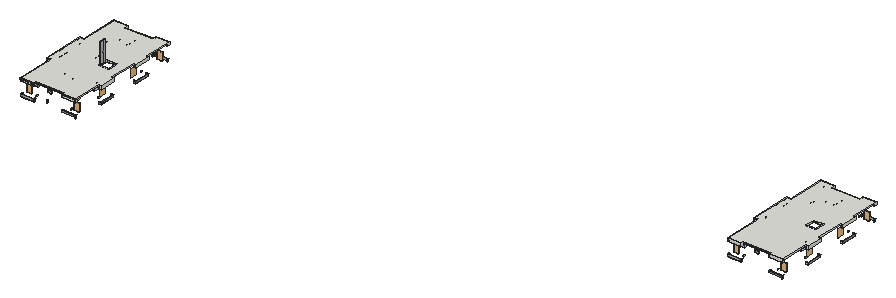
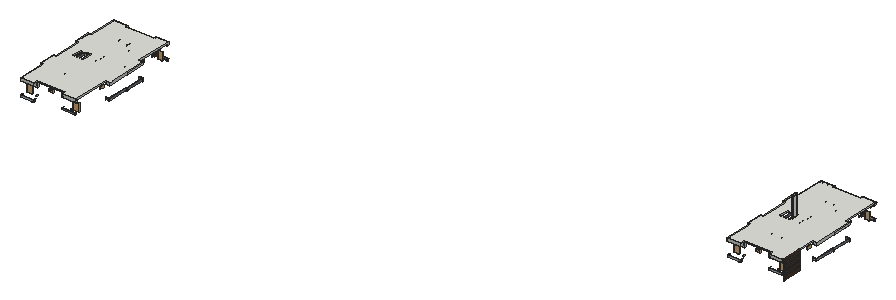
# SketchUp Ruby script. Lengths in inches.
U = 1.inch
M = Sketchup.active_model
def pt(a) = Geom::Point3d.new(a.map { |v| v * U })
def face(e, loops, mat)
  f = e.add_face(loops[0].map { |a| pt(a) })
  loops[1..].each { |l| e.add_face(l.map { |a| pt(a) }).erase! }
  f.material = f.back_material = mat if mat
  f
end
# faces: each face lists its corners as indices into pts; further lists are holes
def faces(e, pts, list, mat = nil) = list.each { |f| face(e, (f[0].is_a?(Array) ? f : [f]).map { |l| l.map { |i| pts[i] } }, mat) }
# xy, xz, yz: faces in a plane at the given z, y or x. An outline is a flat list of corners, or four numbers for a rectangle; further outlines are holes
def ring(l) = l.size == 4 ? [[l[0], l[1]], [l[2], l[1]], [l[2], l[3]], [l[0], l[3]]] : l.each_slice(2).to_a
def flat(e, list, mat, &to3) = list.each { |f| face(e, (f[0].is_a?(Array) ? f : [f]).map { |l| ring(l).map { |u, v| to3.(u, v) } }, mat) }
def xy(e, z, list, mat = nil) = flat(e, list, mat) { |x, y| [x, y, z] }
def xz(e, y, list, mat = nil) = flat(e, list, mat) { |x, z| [x, y, z] }
def yz(e, x, list, mat = nil) = flat(e, list, mat) { |y, z| [x, y, z] }
def lines(e, pts, list) = list.each { |a, b| e.add_line(pt(pts[a]), pt(pts[b])) }
# prism: a flat outline (further loops are holes) pulled along v
def prism(e, loops, v, mat = nil)
  f = face(e, loops, mat); d = Geom::Vector3d.new(v.map { |x| x * U })
  f.pushpull(f.normal.samedirection?(d) ? d.length : -d.length)
end
def box(e, o, s, mat = nil) = prism(e, [[o, [o[0] + s[0], o[1], o[2]], [o[0] + s[0], o[1] + s[1], o[2]], [o[0], o[1] + s[1], o[2]]]], [0, 0, s[2]], mat)
def at(x, y, z, deg = 0) = Geom::Transformation.translation(pt([x, y, z])) * Geom::Transformation.rotation(ORIGIN, Z_AXIS, deg.degrees)
def axes(o, x, y, z) = Geom::Transformation.new([*x, 0, *y, 0, *z, 0, *pt(o).to_a, 1])
def part(name) = M.definitions.add(name)
# library, detail: a bought-in or finely detailed component or shape, given as its bounding box
def library(name, o, s) = part(name).tap { |d| box(d.entities, o, s) }
def detail(e, o, s) = box(e.add_group.entities, o, s)
def put(e, d, t, mat = nil) = e.add_instance(d, t).tap { |i| i.material = mat if mat }
def group(e, t, mat = nil) = e.add_group.tap { |g| g.transformation = t; g.material = mat if mat }.entities
root = M.entities
M.materials.add("0-SS4").color = [255, 255, 255]
M.materials.add("0-SS7").color = [192, 192, 192]
M.materials.add("0-grey 3").color = [204, 204, 204]
M.materials.add("0-off white").color = [255, 255, 255]
M.materials.add("2121 AP  X165 Dhaani-I").color = [217, 210, 92]
M.materials.add("Glass_Basic_01").color = [161, 173, 186]
M.materials["Glass_Basic_01"].alpha = 0.59
M.materials.add("M09_Shadow_Night").color = [0, 0, 0]
M.materials.add("Marble_06_1K").color = [165, 150, 147]
M.materials.add("Wood_Veneer_15_1K").color = [103, 69, 45]
M.materials.add("[0056_Yellow]").color = [255, 255, 0]
c1 = part("Group\#116")
xy(c1.entities,0,[[24,0,24.75,24.75]])
xy(c1.entities,107,[[24,0,24.75,24.75]])
xz(c1.entities,0,[[24,0,24.75,107]])
xz(c1.entities,24.75,[[24,0,24.75,107]])
yz(c1.entities,24,[[0,0,24.75,6],[0,6,24.75,12],[0,12,24.75,18],[0,18,24.75,24],[0,24,24.75,30],
  [0,30,24.75,36],[0,36,24.75,42],[0,42,24.75,48],[0,48,24.75,54],[0,54,24.75,60],
  [0,60,24.75,66],[0,66,24.75,72],[0,72,24.75,78],[0,78,24.75,84],[0,84,24.75,90],
  [0,90,24.75,96],[0,96,24.75,107]],"Wood_Veneer_15_1K")
yz(c1.entities,24.75,[[0,0,24.75,107]])
c2 = part("Group\#85")
xy(c2.entities,0,[[0,0,0,11.0625,2,11.0625,2,2,80,2,80,0],[80,0,82,2],[80,2,82,11.0625]])
xy(c2.entities,16,[[0,0,80,0,80,2,2,2,2,11.0625,0,11.0625],[80,0,82,2],[80,2,82,11.0625]],"M09_Shadow_Night")
xz(c2.entities,0,[[80,0,82,16]])
xz(c2.entities,0,[[0,0,80,16]],"Glass_Basic_01")
xz(c2.entities,2,[[2,0,80,16],[80,0,82,16]])
xz(c2.entities,11.0625,[[0,0,2,16],[80,0,82,16]])
yz(c2.entities,0,[[0,0,11.0625,16]])
yz(c2.entities,2,[[2,0,11.0625,16]])
yz(c2.entities,80,[[0,0,2,16],[2,0,11.0625,16]])
yz(c2.entities,82,[[0,0,2,16],[2,0,11.0625,16]])
c3 = part("Group\#90")
xy(c3.entities,0,[[0,0,0,11.0625,2,11.0625,2,2,80,2,80,0],[80,0,82,2],[80,2,82,11.0625]])
xy(c3.entities,16,[[0,0,80,0,80,2,2,2,2,11.0625,0,11.0625],[80,0,82,2],[80,2,82,11.0625]],"M09_Shadow_Night")
xz(c3.entities,0,[[80,0,82,16]])
xz(c3.entities,0,[[0,0,80,16]],"Glass_Basic_01")
xz(c3.entities,2,[[2,0,80,16],[80,0,82,16]])
xz(c3.entities,11.0625,[[0,0,2,16],[80,0,82,16]])
yz(c3.entities,0,[[0,0,11.0625,16]])
yz(c3.entities,2,[[2,0,11.0625,16]])
yz(c3.entities,80,[[0,0,2,16],[2,0,11.0625,16]])
yz(c3.entities,82,[[0,0,2,16],[2,0,11.0625,16]])
c4 = part("Group\#86")
xy(c4.entities,0,[[80,-8.86,82,2],[2,0,80,2]])
xy(c4.entities,16,[[80,-8.86,82,2],[2,0,80,2]],"M09_Shadow_Night")
xz(c4.entities,-8.86,[[80,0,82,16]],"M09_Shadow_Night")
xz(c4.entities,0,[[2,0,80,16]],"Glass_Basic_01")
xz(c4.entities,2,[[2,0,80,16]])
yz(c4.entities,2,[[0,0,2,16]],"M09_Shadow_Night")
yz(c4.entities,80,[[-8.86,0,0,16],[0,0,2,16]])
yz(c4.entities,82,[[-8.86,0,2,16]])
c5 = part("Group\#87")
xy(c5.entities,0,[[0,0,0,11.0625,2,11.0625,2,2,80,2,80,0],[80,0,82,2],[80,2,82,11.0625]])
xy(c5.entities,16,[[0,0,80,0,80,2,2,2,2,11.0625,0,11.0625],[80,0,82,2],[80,2,82,11.0625]],"M09_Shadow_Night")
xz(c5.entities,0,[[0,0,80,16]],"Glass_Basic_01")
xz(c5.entities,0,[[80,0,82,16]],"M09_Shadow_Night")
xz(c5.entities,2,[[2,0,80,16],[80,0,82,16]])
xz(c5.entities,11.0625,[[0,0,2,16],[80,0,82,16]])
yz(c5.entities,0,[[0,0,11.0625,16]])
yz(c5.entities,2,[[2,0,11.0625,16]])
yz(c5.entities,80,[[0,0,2,16],[2,0,11.0625,16]])
yz(c5.entities,82,[[2,0,11.0625,16]])
yz(c5.entities,82,[[0,0,2,16]],"M09_Shadow_Night")
c6 = part("Group\#89")
xy(c6.entities,0,[[0,0,0,11.0625,2,11.0625,2,2,80,2,80,0],[80,0,82,2],[80,2,82,11.0625]])
xy(c6.entities,16,[[0,0,80,0,80,2,2,2,2,11.0625,0,11.0625],[80,0,82,2],[80,2,82,11.0625]],"M09_Shadow_Night")
xz(c6.entities,0,[[0,0,80,16]],"Glass_Basic_01")
xz(c6.entities,0,[[80,0,82,16]],"M09_Shadow_Night")
xz(c6.entities,2,[[2,0,80,16],[80,0,82,16]])
xz(c6.entities,11.0625,[[0,0,2,16],[80,0,82,16]])
yz(c6.entities,0,[[0,0,11.0625,16]])
yz(c6.entities,2,[[2,0,11.0625,16]])
yz(c6.entities,80,[[0,0,2,16],[2,0,11.0625,16]])
yz(c6.entities,82,[[2,0,11.0625,16]])
yz(c6.entities,82,[[0,0,2,16]],"M09_Shadow_Night")
c7 = part("Group\#88")
xy(c7.entities,0,[[2,0,80,2],[80,0,82,2],[80,2,82,11.0625]])
xy(c7.entities,16,[[2,0,80,2],[80,0,82,2],[80,2,82,11.0625]],"M09_Shadow_Night")
xz(c7.entities,0,[[2,0,80,16]],"Glass_Basic_01")
xz(c7.entities,0,[[80,0,82,16]],"M09_Shadow_Night")
xz(c7.entities,2,[[2,0,80,16],[80,0,82,16]])
xz(c7.entities,11.0625,[[80,0,82,16]],"M09_Shadow_Night")
yz(c7.entities,2,[[0,0,2,16]],"M09_Shadow_Night")
yz(c7.entities,80,[[0,0,2,16],[2,0,11.0625,16]])
yz(c7.entities,82,[[2,0,11.0625,16]])
yz(c7.entities,82,[[0,0,2,16]],"M09_Shadow_Night")
c8 = library("Slide Window 5'",[0,-2.02,0],[60,2.02,54])
c9 = library("Group\#52",[0,0,0],[4.66,6.14,3.22])
c10 = part("Wall light")
xy(c10.entities,0,[[1.3,1.93,0.875,2.1,0.51,2.38,0.23,2.74,0.06,3.17,0,3.62,0.06,4.07,0.23,4.49,0.51,4.86,0.875,5.13,1.3,5.31,1.75,5.37,2.2,5.31,2.625,5.13,2.99,4.86,3.27,4.49,3.44,4.07,3.5,3.62,3.44,3.17,3.27,2.74,2.99,2.38,2.625,2.1,2.2,1.93]],"[0056_Yellow]")
xy(c10.entities,0.74,[[1.01,0,2.57,1.93]])
xy(c10.entities,10.13,[[1.01,0,2.57,0,2.57,1.93,2.2,1.93,1.75,1.87,1.3,1.93,1.01,1.93]])
xy(c10.entities,10.875,[[1.75,1.87,2.2,1.93,1.3,1.93]])
xy(c10.entities,10.875,[[1.3,1.93,2.2,1.93,2.625,2.1,2.99,2.38,3.27,2.74,3.44,3.17,3.5,3.62,3.44,4.07,3.27,4.49,2.99,4.86,2.625,5.13,2.2,5.31,1.75,5.37,1.3,5.31,0.875,5.13,0.51,4.86,0.23,4.49,0.06,4.07,0,3.62,0.06,3.17,0.23,2.74,0.51,2.38,0.875,2.1]],"[0056_Yellow]")
xz(c10.entities,0,[[1.01,0.74,2.57,10.13]])
xz(c10.entities,1.93,[[1.3,0,2.2,0.74],[1.01,0.74,1.3,10.13],[1.3,0.74,2.2,10.875],[2.2,0.74,2.57,10.13]])
yz(c10.entities,1.01,[[0,0.74,1.93,10.13]])
yz(c10.entities,2.57,[[0,0.74,1.93,10.13]])
p = [[1.3,1.93,10.875],[0.875,2.1,10.875],[0.875,2.1,0],[1.3,1.93,0],[1.3,1.93,0.74],[1.3,1.93,10.13],
  [2.625,2.1,10.875],[2.2,1.93,10.875],[2.2,1.93,10.13],[2.2,1.93,0.74],[2.2,1.93,0],[2.625,2.1,0],
  [0.51,2.38,10.875],[0.51,2.38,0],[2.99,2.38,10.875],[2.99,2.38,0],[0.23,2.74,10.875],[0.23,2.74,0],
  [3.27,2.74,10.875],[3.27,2.74,0],[0.06,3.17,10.875],[0.06,3.17,0],[3.44,3.17,10.875],[3.44,3.17,0],
  [0,3.62,10.875],[0,3.62,0],[3.5,3.62,10.875],[3.5,3.62,0],[0.06,4.07,10.875],[0.06,4.07,0],
  [3.44,4.07,10.875],[3.44,4.07,0],[0.23,4.49,10.875],[0.23,4.49,0],[3.27,4.49,10.875],[3.27,4.49,0],
  [0.51,4.86,10.875],[0.51,4.86,0],[2.99,4.86,10.875],[2.99,4.86,0],[0.875,5.13,10.875],[0.875,5.13,0],
  [2.625,5.13,10.875],[2.625,5.13,0],[1.3,5.31,10.875],[1.3,5.31,0],[2.2,5.31,10.875],[2.2,5.31,0],
  [1.75,5.37,10.875],[1.75,5.37,0],[1.75,1.87,10.875],[1.75,1.87,10.13]]
faces(c10.entities,p,[[0,1,2,3,4,5],[6,7,8,9,10,11],[1,12,13,2],[14,6,11,15],[12,16,17,13],[18,14,15,19],[16,20,21,17],[22,18,19,23],
  [20,24,25,21],[26,22,23,27],[24,28,29,25],[30,26,27,31],[28,32,33,29],[34,30,31,35],[32,36,37,33],[38,34,35,39],
  [36,40,41,37],[42,38,39,43],[40,44,45,41],[46,42,43,47],[44,48,49,45],[48,46,47,49],[50,0,5,51],[7,50,51,8]])
c11 = part("Group\#305")
xy(c11.entities,0.81,[[0.28,-0.04,1.69,0]],"0-off white")
xz(c11.entities,-0.04,[[0.28,0.81,1.69,0.81,0.98,1.5]],"0-off white")
xz(c11.entities,0,[[[0.98,0,1.24,0.03,1.48,0.13,1.68,0.29,1.84,0.49,1.93,0.73,1.97,0.98,1.93,1.24,1.84,1.48,1.68,1.68,1.48,1.84,1.24,1.93,0.98,1.97,0.73,1.93,0.49,1.84,0.29,1.68,0.13,1.48,0.03,1.24,0,0.98,0.03,0.73,0.13,0.49,0.29,0.29,0.49,0.13,0.73,0.03],[0.28,0.81,0.98,1.5,1.69,0.81]]],"0-off white")
xz(c11.entities,0.63,[[0.98,0,0.73,0.03,0.49,0.13,0.29,0.29,0.13,0.49,0.03,0.73,0,0.98,0.03,1.24,0.13,1.48,0.29,1.68,0.49,1.84,0.73,1.93,0.98,1.97,1.24,1.93,1.48,1.84,1.68,1.68,1.84,1.48,1.93,1.24,1.97,0.98,1.93,0.73,1.84,0.49,1.68,0.29,1.48,0.13,1.24,0.03]],"0-off white")
p = [[0.49,0.63,0.13],[0.73,0.63,0.03],[0.73,0,0.03],[0.49,0,0.13],[0.98,0.63,0],[0.98,0,0],
  [1.24,0.63,0.03],[1.24,0,0.03],[1.48,0.63,0.13],[1.48,0,0.13],[0.29,0.63,0.29],[0.29,0,0.29],
  [1.68,0.63,0.29],[1.68,0,0.29],[0.13,0.63,0.49],[0.13,0,0.49],[1.84,0.63,0.49],[1.84,0,0.49],
  [0.03,0.63,0.73],[0.03,0,0.73],[1.93,0.63,0.73],[1.93,0,0.73],[0,0.63,0.98],[0,0,0.98],
  [1.97,0.63,0.98],[1.97,0,0.98],[0.98,0,1.5],[0.28,0,0.81],[0.28,-0.04,0.81],[0.98,-0.04,1.5],
  [1.69,0,0.81],[1.69,-0.04,0.81],[0.03,0.63,1.24],[0.03,0,1.24],[1.93,0.63,1.24],[1.93,0,1.24],
  [0.13,0.63,1.48],[0.13,0,1.48],[1.84,0.63,1.48],[1.84,0,1.48],[0.29,0.63,1.68],[0.29,0,1.68],
  [1.68,0.63,1.68],[1.68,0,1.68],[0.49,0.63,1.84],[0.49,0,1.84],[1.48,0.63,1.84],[1.48,0,1.84],
  [0.73,0.63,1.93],[0.73,0,1.93],[1.24,0.63,1.93],[1.24,0,1.93],[0.98,0.63,1.97],[0.98,0,1.97]]
faces(c11.entities,p,[[0,1,2,3],[1,4,5,2],[4,6,7,5],[6,8,9,7],[10,0,3,11],[8,12,13,9],[14,10,11,15],[12,16,17,13],
  [18,14,15,19],[16,20,21,17],[22,18,19,23],[20,24,25,21],[26,27,28,29],[30,26,29,31],[32,22,23,33],[24,34,35,25],
  [36,32,33,37],[34,38,39,35],[40,36,37,41],[38,42,43,39],[44,40,41,45],[42,46,47,43],[48,44,45,49],[46,50,51,47],
  [52,48,49,53],[50,52,53,51]],"0-off white")
c12 = part("Group\#370")
box(c12.entities,[0,0,-0.39],[5.12,10.31,0.39])
g1 = group(c12.entities,at(1.59,1.64,0.22))
put(g1,c11,axes([0,4.49,0],[1,0,0],[0,0,-0.35294],[0,1,0]))
put(g1,c11,axes([0,2,0],[1,0,0],[0,0,-0.35294],[0,-1,0]))
c13 = library("Group\#46",[0,-0.05,0],[30,2.55,24])
c14 = library("Group\#115",[0,0,0],[72,16,6.2])
c15 = part("Group\#111")
xy(c15.entities,-36.67,[[252.4,-12,252.4,0,259.49,0,259.49,-8,330.4,-8,330.4,0,336.4,0,336.4,-12]])
xy(c15.entities,-36.53,[[0,-12,0,-0.08,6,-0.08,6,-8,78,-8,78,0,84,0,84,-12],[336.4,163,336.4,169,349.41,169,349.41,255,336.4,255,336.4,261,353.41,261,353.41,163],[-24,217,-24,336.57,-20,336.57,-20,222,0,222,0,217],[-24,342.21,-24,473,0,473,0,468,-20,468,-20,342.21],[336.4,430,336.4,435,347.875,435,347.875,523,335.62,523,335.62,528,351.875,528,351.875,430],
  [0,689.93,0,701.93,84,701.93,84,689.93,78,689.93,78,697.93,6,697.93,6,689.93],[252.4,689.93,252.4,701.93,336.4,701.93,336.4,689.93,330.4,689.93,330.4,697.93,258.4,697.93,258.4,689.93]])
xy(c15.entities,-24.53,[[[6,-8,6,-0.08,0,-0.08,0,222,-20,222,-20,336.57,-24,336.57,-24,342.21,-20,342.21,-20,468,0,468,0,689.93,6,689.93,6,697.93,78,697.93,78,689.93,84,689.93,84,678,252.4,678,252.4,689.93,258.4,689.93,258.4,697.93,330.4,697.93,330.4,689.93,336.4,689.93,336.4,528,335.62,528,335.62,523,347.875,523,347.875,435,336.4,435,336.4,255,349.41,255,349.41,169,336.4,169,336.4,0,330.4,0,330.4,-8,259.49,-8,259.49,0,78,0,78,-8],[216.4,315,276.4,375]],[-24,217,0,217,0,222,-20,222,-20,336.57,-24,336.57]])
xy(c15.entities,-18.53,[[[0,-12,84,-12,84,0,252.4,0,252.4,-12,336.4,-12,336.4,163,353.41,163,353.41,261,336.4,261,336.4,430,351.875,430,351.875,528,336.4,528,336.4,701.93,252.4,701.93,252.4,678,84,678,84,701.93,0,701.93,0,473,-24,473,-24,217,0,217],[216.4,315,276.4,375]]])
xz(c15.entities,-12,[[252.4,-36.67,336.4,-18.53],[0,-36.53,84,-18.53]])
xz(c15.entities,-8,[[259.49,-36.67,330.4,-24.53],[6,-36.53,78,-24.53]])
xz(c15.entities,-0.08,[[0,-36.53,6,-24.53]])
xz(c15.entities,0,[[252.4,-36.67,259.49,-24.53],[330.4,-36.67,336.4,-24.53],[78,-36.53,84,-24.53],[84,-24.53,252.4,-18.53]])
xz(c15.entities,163,[[336.4,-36.53,353.41,-18.53]])
xz(c15.entities,169,[[336.4,-36.53,349.41,-24.53]])
xz(c15.entities,217,[[-24,-36.53,0,-24.53],[-24,-24.53,0,-18.53]])
xz(c15.entities,222,[[-20,-36.53,0,-24.53]])
xz(c15.entities,255,[[336.4,-36.53,349.41,-24.53]])
xz(c15.entities,261,[[336.4,-36.53,353.41,-18.53]])
xz(c15.entities,315,[[216.4,-24.53,276.4,-18.53]])
xz(c15.entities,336.57,[[-24,-36.53,-20,-24.53]])
xz(c15.entities,342.21,[[-24,-36.53,-20,-24.53]])
xz(c15.entities,375,[[216.4,-24.53,276.4,-18.53]])
xz(c15.entities,430,[[336.4,-36.53,351.875,-18.53]])
xz(c15.entities,435,[[336.4,-36.53,347.875,-24.53]])
xz(c15.entities,468,[[-20,-36.53,0,-24.53]])
xz(c15.entities,473,[[-24,-36.53,0,-18.53]])
xz(c15.entities,523,[[335.62,-36.53,347.875,-24.53]])
xz(c15.entities,528,[[335.62,-36.53,351.875,-24.53],[336.4,-24.53,351.875,-18.53]])
xz(c15.entities,678,[[84,-24.53,252.4,-18.53]])
xz(c15.entities,689.93,[[0,-36.53,6,-24.53],[78,-36.53,84,-24.53],[252.4,-36.53,258.4,-24.53],[330.4,-36.53,336.4,-24.53]])
xz(c15.entities,697.93,[[6,-36.53,78,-24.53],[258.4,-36.53,330.4,-24.53]])
xz(c15.entities,701.93,[[0,-36.53,84,-18.53],[252.4,-36.53,336.4,-18.53]])
yz(c15.entities,-24,[[217,-36.53,336.57,-24.53],[342.21,-36.53,342.21,-24.53,217,-24.53,217,-18.53,473,-18.53,473,-36.53]])
yz(c15.entities,-20,[[222,-36.53,336.57,-24.53],[342.21,-36.53,468,-24.53]])
yz(c15.entities,0,[[-12,-36.53,-12,-18.53,217,-18.53,217,-24.53,-0.08,-24.53,-0.08,-36.53],[217,-36.53,222,-24.53],[468,-36.53,473,-24.53],[689.93,-36.53,701.93,-24.53],[473,-24.53,701.93,-18.53]])
yz(c15.entities,6,[[-8,-36.53,-0.08,-24.53],[689.93,-36.53,697.93,-24.53]])
yz(c15.entities,78,[[-8,-36.53,0,-24.53],[689.93,-36.53,697.93,-24.53]])
yz(c15.entities,84,[[-12,-36.53,0,-18.53],[689.93,-36.53,701.93,-36.53,701.93,-18.53,678,-18.53,678,-24.53,689.93,-24.53]])
yz(c15.entities,216.4,[[315,-24.53,375,-18.53]])
yz(c15.entities,252.4,[[-12,-36.67,0,-18.53],[689.93,-36.53,701.93,-24.53],[678,-24.53,701.93,-18.53]])
yz(c15.entities,258.4,[[689.93,-36.53,697.93,-24.53]])
yz(c15.entities,259.49,[[-8,-36.67,0,-24.53]])
yz(c15.entities,276.4,[[315,-24.53,375,-18.53]])
yz(c15.entities,330.4,[[-8,-36.67,0,-24.53],[689.93,-36.53,697.93,-24.53]])
yz(c15.entities,335.62,[[523,-36.53,528,-24.53]])
yz(c15.entities,336.4,[[-12,-36.67,0,-24.53],[163,-36.53,169,-24.53],[255,-36.53,261,-24.53],[430,-36.53,435,-24.53],[689.93,-36.53,701.93,-36.53,701.93,-18.53,528,-18.53,528,-24.53,689.93,-24.53],
  [-12,-24.53,163,-18.53],[261,-24.53,430,-18.53]])
yz(c15.entities,347.875,[[435,-36.53,523,-24.53]])
yz(c15.entities,349.41,[[169,-36.53,255,-24.53]])
yz(c15.entities,351.875,[[430,-36.53,528,-18.53]])
yz(c15.entities,353.41,[[163,-36.53,261,-18.53]])
c16 = part("Lift Door")
g2 = group(c16.entities,at(22.98,-1.97,0))
xy(g2,0,[[-11.49,0,22.98,1.97]],"0-SS7")
xy(g2,81.69,[[-11.49,0,22.98,1.97]],"0-SS7")
xz(g2,0,[[-11.49,0,22.98,81.69]],"0-SS7")
xz(g2,1.97,[[-11.49,0,22.98,81.69]],"0-SS4")
yz(g2,-11.49,[[0,0,1.97,81.69]],"0-SS7")
yz(g2,22.98,[[0,0,1.97,81.69]],"0-SS7")
c17 = part("Group\#83")
put(c17.entities,c16,axes([5.4,10.39,0],[0,0.42899,0],[-0.53123,0,0],[0,0,1.07229]),"0-grey 3")
put(c17.entities,c16,axes([5.4,-4.4,0],[0,0.42899,0],[-0.53123,0,0],[0,0,1.07229]),"0-grey 3")
g3 = group(c17.entities,at(0,44.39,0))
p = [[0,-44.39,88.58],[0,-13.75,88.58],[0,-13.75,0],[0,-44.39,0]]
lines(g3,p,[[0,1],[1,2],[3,0],[2,3]])
g4 = group(c17.entities,at(2.42,30.63,0))
prism(g4,[[[2.98,-30.63,0],[2.98,-30.11,0],[2.98,-30.11,87.6],[2.98,-0.53,87.6],[2.98,-0.53,0],[2.98,0,0],[2.98,0,88.58],[2.98,-30.63,88.58]]],[-5.4,0,0])
box(root,[3718.46,1104.875,329.9375],[6,30,36])
box(root,[119.8,217.34,329.9375],[6,30,36])
box(root,[3672.46,1596.875,330],[30,6,36])
box(root,[3930.84,1428.875,330],[6.02,30,36])
box(root,[3636.46,1292.43,330],[6,71.13,36])
box(root,[3882.86,1596.875,330],[30,6,36])
box(root,[3780.46,1279.09,330],[6,48,36])
box(root,[3718.46,1428.875,330],[6,30,36])
box(root,[3816.86,1518.875,330],[6,30,36])
box(root,[3930.86,1104.875,330],[6,30,36])
box(root,[3636.46,1182.875,330],[6,72,36])
box(root,[3882.86,960.875,330],[30,6,36])
box(root,[3780.46,1225.09,330],[6,48.35,36])
box(root,[3674.86,960.875,330],[27.6,6,36])
box(root,[3762.46,1470.875,330],[6,42,36])
box(root,[3816.86,1470.875,330],[6,42,36])
box(root,[3816.86,1050.875,330],[6,42,36])
box(root,[3816.86,1014.875,330],[6,30,36])
box(root,[3762.46,1050.875,330],[6,38.53,36])
box(root,[284.2,709.34,330],[30,6,36])
box(root,[37.8,404.89,330],[6,71.14,36],"Marble_06_1K")
box(root,[332.19,541.34,330],[6.01,30,36])
box(root,[119.8,541.34,330],[6,30,36])
box(root,[218.2,631.34,330],[6,30,36])
box(root,[332.2,217.34,330],[6,30,36])
box(root,[181.8,391.55,330],[6,48,36])
box(root,[181.8,337.55,330],[6,48.35,36])
box(root,[76.2,73.34,330],[27.6,6,36],"Marble_06_1K")
box(root,[218.2,127.34,330],[6,30,36])
box(root,[218.2,583.34,330],[6,42,36])
box(root,[218.2,163.34,330],[6,42,36])
box(root,[163.8,583.34,330],[6,42,36])
box(root,[163.8,163.34,330],[6,38.53,36])
box(root,[73.8,709.34,330],[30,6,36])
xy(root,330,[[284.2,73.34,314.2,79.34],[37.8,295.34,43.8,367.34]])
xy(root,366,[[284.2,73.34,314.2,79.34],[37.8,295.34,43.8,367.34]])
xz(root,73.34,[[284.2,330,314.2,366]],"Marble_06_1K")
xz(root,79.34,[[284.2,330,314.2,366]])
xz(root,295.34,[[37.8,330,43.8,366]])
xz(root,367.34,[[37.8,330,43.8,366]])
yz(root,37.8,[[295.34,330,367.34,366]],"Marble_06_1K")
yz(root,43.8,[[295.34,330,367.34,366]])
yz(root,284.2,[[73.34,330,79.34,366]])
yz(root,314.2,[[73.34,330,79.34,366]])
p = [[108.8,38.27,266],[28.8,38.27,266],[106.8,40.27,266],[106.8,49.34,266],[108.8,49.34,266],[28.8,40.27,266],
  [3705.46,927.8125,266],[3705.46,936.875,266],[3707.46,925.8125,266],[3707.46,936.875,266],[3627.46,927.8125,266],[3627.46,925.8125,266]]
lines(root,p,[[0,1],[2,3],[0,4],[5,2],[6,7],[8,9],[10,6],[8,11]])
put(root,c1,axes([1.05,618.07,252],[1,0,0],[0,4.89695,0],[0,0,1.1215]),"Wood_Veneer_15_1K")
put(root,c2,axes([3976.33,1366.875,264],[0,1.18,0],[-1.39867,0,0],[0,0,1]),"Glass_Basic_01")
put(root,c3,at(3959.86,1637.87,264,180),"Glass_Basic_01")
put(root,c2,axes([377.67,479.34,264],[0,1.18,0],[-1.39867,0,0],[0,0,1]),"Glass_Basic_01")
put(root,c3,at(361.2,750.33,264,180),"Glass_Basic_01")
put(root,c2,axes([3977.86,1099.875,266],[0,1.18,0],[-1.537,0,0],[0,0,1]),"Glass_Basic_01")
put(root,c4,axes([3605.56,1275.82,266],[0,1.63485,0],[-2.08447,0,0],[0,0,1]),"Glass_Basic_01")
put(root,c5,at(3625.46,925.8125,266),"Glass_Basic_01")
put(root,c6,at(3877.86,925.8125,266),"Glass_Basic_01")
put(root,c7,axes([3601.4,1276.05,266],[0,-1.49,0],[2.08447,0,0],[0,0,1]),"Glass_Basic_01")
put(root,c2,axes([379.2,212.34,266],[0,1.18,0],[-1.537,0,0],[0,0,1]),"Glass_Basic_01")
put(root,c5,at(26.8,38.27,266),"Glass_Basic_01")
put(root,c4,axes([6.91,388.28,266],[0,1.63485,0],[-2.08447,0,0],[0,0,1]),"Glass_Basic_01")
put(root,c6,at(279.2,38.27,266),"Glass_Basic_01")
put(root,c7,axes([2.74,388.52,266],[0,-1.49,0],[2.08447,0,0],[0,0,1]),"Glass_Basic_01")
put(root,c8,axes([3935.68,1179.88,281.33],[0,-0.65004,0],[1.4091,0,0],[0,0,0.88889]))
put(root,c8,axes([337.02,292.34,281.33],[0,-0.65004,0],[1.4091,0,0],[0,0,0.88889]))
put(root,c8,axes([3935.59,1416.93,281.94],[0,-0.65094,0],[1.4091,0,0],[0,0,0.88889]))
put(root,c8,axes([336.93,529.39,281.94],[0,-0.65094,0],[1.4091,0,0],[0,0,0.88889]))
put(root,c8,axes([3662.86,962.66,282],[-0.49488,0,0],[0,-1.4091,0],[0,0,0.89778]))
put(root,c8,axes([64.2,75.12,282],[-0.49488,0,0],[0,-1.4091,0],[0,0,0.89778]))
put(root,c8,axes([3632.46,1600.77,282],[0.63333,0,0],[0,1.4091,0],[0,0,0.88889]))
put(root,c8,axes([3914.86,1600.6875,282],[0.63333,0,0],[0,1.4091,0],[0,0,0.88889]))
put(root,c8,axes([3953.86,962.66,282],[-0.58385,0,0],[0,-1.4091,0],[0,0,0.88889]))
put(root,c3,at(3707.46,1637.87,282,180),"Glass_Basic_01")
put(root,c8,axes([33.8,713.23,282],[0.63333,0,0],[0,1.4091,0],[0,0,0.88889]))
put(root,c8,axes([355.2,75.12,282],[-0.58385,0,0],[0,-1.4091,0],[0,0,0.88889]))
put(root,c8,axes([316.2,713.15,282],[0.63333,0,0],[0,1.4091,0],[0,0,0.88889]))
put(root,c3,at(108.8,750.33,282,180),"Glass_Basic_01")
put(root,c9,at(3700.46,962.59,282.64,180))
put(root,c9,at(101.8,75.06,282.64,180))
put(root,c9,at(3886.29,1601.16,282.75))
put(root,c9,at(3935.14,1132.69,282.75,-90))
put(root,c9,at(3935.14,1456.875,282.75,-90))
put(root,c9,at(336.48,245.16,282.75,-90))
put(root,c9,at(336.48,569.34,282.75,-90))
put(root,c9,at(287.63,713.62,282.75))
put(root,c9,at(3673.74,1601.34,282.89))
put(root,c9,at(75.08,713.8,282.89))
put(root,c9,at(3910.86,960.875,284.0625,180))
put(root,c9,at(312.2,73.34,284.0625,180))
put(root,c10,axes([185.97,49.34,287],[-1.35,0,0],[0,-1.35,0],[0,0,1.35]))
put(root,c12,axes([3834.86,1309.47,296.05],[0,-0.53664,0],[0,0,1],[-1.59369,0,0]))
put(root,c12,axes([236.2,421.93,296.05],[0,-0.53664,0],[0,0,1],[-1.59369,0,0]))
put(root,c13,axes([3625.26,1446.875,342],[0,-0.8,0],[1.27878,0,0],[0,0,0.5]))
put(root,c13,axes([3804.86,1613.09,342],[-0.81341,0,0],[0,-1.27878,0],[0,0,0.5]))
put(root,c13,axes([3625.26,1140.875,342],[0,-0.8,0],[1.27878,0,0],[0,0,0.5]))
put(root,c13,axes([206.2,725.55,342],[-0.81341,0,0],[0,-1.27878,0],[0,0,0.5]))
put(root,c13,axes([26.6,253.34,342],[0,-0.8,0],[1.27878,0,0],[0,0,0.5]))
put(root,c13,axes([26.6,559.34,342],[0,-0.8,0],[1.27878,0,0],[0,0,0.5]))
put(root,c13,axes([3780.46,937.56,342],[0.81333,0,0],[0,1.27878,0],[0,0,0.5]))
put(root,c13,axes([181.8,50.02,342],[0.81333,0,0],[0,1.27878,0],[0,0,0.5]))
put(root,c14,axes([5.8,385.9,359.5],[0,-1.5912,0],[2,0,0],[0,0,-1]))
put(root,c14,axes([285.28,41.34,359.86],[1,0,0],[0,2,0],[0,0,-1]))
put(root,c14,axes([31.8,41.34,360],[1,0,0],[0,2,0],[0,0,-1]))
put(root,c15,at(3624.46,936.95,390.53))
g5 = group(root,at(25.8,49.34,390.53))
xy(g5,-36.67,[[252.4,-12,252.4,0,259.49,0,259.49,-8,330.4,-8,330.4,0,336.4,0,336.4,-12]])
xy(g5,-36.53,[[0,-12,0,-0.08,6,-0.08,6,-8,78,-8,78,0,84,0,84,-12],[336.4,163,336.4,169,349.41,169,349.41,255,336.4,255,336.4,261,353.41,261,353.41,163],[-24,217,-24,336.57,-20,336.57,-20,222,0,222,0,217],[-24,342.21,-24,473,0,473,0,468,-20,468,-20,342.21],[336.4,430,336.4,435,347.875,435,347.875,523,335.62,523,335.62,528,351.875,528,351.875,430],
  [0,689.93,0,701.93,84,701.93,84,689.93,78,689.93,78,697.93,6,697.93,6,689.93],[252.4,689.93,252.4,701.93,336.4,701.93,336.4,689.93,330.4,689.93,330.4,697.93,258.4,697.93,258.4,689.93]])
xy(g5,-24.53,[[[6,-8,6,-0.08,0,-0.08,0,222,-20,222,-20,336.57,-24,336.57,-24,342.21,-20,342.21,-20,468,0,468,0,689.93,6,689.93,6,697.93,78,697.93,78,689.93,84,689.93,84,678,252.4,678,252.4,689.93,258.4,689.93,258.4,697.93,330.4,697.93,330.4,689.93,336.4,689.93,336.4,528,335.62,528,335.62,523,347.875,523,347.875,435,336.4,435,336.4,255,349.41,255,349.41,169,336.4,169,336.4,0,330.4,0,330.4,-8,259.49,-8,259.49,0,78,0,78,-8],[216.4,315,276.4,375]],[-24,217,0,217,0,222,-20,222,-20,336.57,-24,336.57]])
xy(g5,-18.53,[[[0,-12,84,-12,84,0,252.4,0,252.4,-12,336.4,-12,336.4,163,353.41,163,353.41,261,336.4,261,336.4,430,351.875,430,351.875,528,336.4,528,336.4,701.93,252.4,701.93,252.4,678,84,678,84,701.93,0,701.93,0,473,-24,473,-24,217,0,217],[216.4,315,276.4,375]]])
xz(g5,-12,[[252.4,-36.67,336.4,-18.53],[0,-36.53,84,-18.53]])
xz(g5,-8,[[259.49,-36.67,330.4,-24.53],[6,-36.53,78,-24.53]])
xz(g5,-0.08,[[0,-36.53,6,-24.53]])
xz(g5,0,[[252.4,-36.67,259.49,-24.53],[330.4,-36.67,336.4,-24.53],[78,-36.53,84,-24.53],[84,-24.53,252.4,-18.53]])
xz(g5,163,[[336.4,-36.53,353.41,-18.53]])
xz(g5,169,[[336.4,-36.53,349.41,-24.53]])
xz(g5,217,[[-24,-36.53,0,-24.53],[-24,-24.53,0,-18.53]])
xz(g5,222,[[-20,-36.53,0,-24.53]])
xz(g5,255,[[336.4,-36.53,349.41,-24.53]])
xz(g5,261,[[336.4,-36.53,353.41,-18.53]])
xz(g5,315,[[216.4,-24.53,276.4,-18.53]])
xz(g5,336.57,[[-24,-36.53,-20,-24.53]])
xz(g5,342.21,[[-24,-36.53,-20,-24.53]])
xz(g5,375,[[216.4,-24.53,276.4,-18.53]])
xz(g5,430,[[336.4,-36.53,351.875,-18.53]])
xz(g5,435,[[336.4,-36.53,347.875,-24.53]])
xz(g5,468,[[-20,-36.53,0,-24.53]])
xz(g5,473,[[-24,-36.53,0,-18.53]])
xz(g5,523,[[335.62,-36.53,347.875,-24.53]])
xz(g5,528,[[335.62,-36.53,351.875,-24.53],[336.4,-24.53,351.875,-18.53]])
xz(g5,678,[[84,-24.53,252.4,-18.53]])
xz(g5,689.93,[[0,-36.53,6,-24.53],[78,-36.53,84,-24.53],[252.4,-36.53,258.4,-24.53],[330.4,-36.53,336.4,-24.53]])
xz(g5,697.93,[[6,-36.53,78,-24.53],[258.4,-36.53,330.4,-24.53]])
xz(g5,701.93,[[0,-36.53,84,-18.53],[252.4,-36.53,336.4,-18.53]])
yz(g5,-24,[[217,-36.53,336.57,-24.53],[342.21,-36.53,342.21,-24.53,217,-24.53,217,-18.53,473,-18.53,473,-36.53]])
yz(g5,-20,[[222,-36.53,336.57,-24.53],[342.21,-36.53,468,-24.53]])
yz(g5,0,[[-12,-36.53,-12,-18.53,217,-18.53,217,-24.53,-0.08,-24.53,-0.08,-36.53],[217,-36.53,222,-24.53],[468,-36.53,473,-24.53],[689.93,-36.53,701.93,-24.53],[473,-24.53,701.93,-18.53]])
yz(g5,6,[[-8,-36.53,-0.08,-24.53],[689.93,-36.53,697.93,-24.53]])
yz(g5,78,[[-8,-36.53,0,-24.53],[689.93,-36.53,697.93,-24.53]])
yz(g5,84,[[-12,-36.53,0,-18.53],[689.93,-36.53,701.93,-36.53,701.93,-18.53,678,-18.53,678,-24.53,689.93,-24.53]])
yz(g5,216.4,[[315,-24.53,375,-18.53]])
yz(g5,252.4,[[-12,-36.67,0,-18.53],[689.93,-36.53,701.93,-24.53],[678,-24.53,701.93,-18.53]])
yz(g5,258.4,[[689.93,-36.53,697.93,-24.53]])
yz(g5,259.49,[[-8,-36.67,0,-24.53]])
yz(g5,276.4,[[315,-24.53,375,-18.53]])
yz(g5,330.4,[[-8,-36.67,0,-24.53],[689.93,-36.53,697.93,-24.53]])
yz(g5,335.62,[[523,-36.53,528,-24.53]])
yz(g5,336.4,[[-12,-36.67,0,-24.53],[163,-36.53,169,-24.53],[255,-36.53,261,-24.53],[430,-36.53,435,-24.53],[689.93,-36.53,701.93,-36.53,701.93,-18.53,528,-18.53,528,-24.53,689.93,-24.53],
  [-12,-24.53,163,-18.53],[261,-24.53,430,-18.53]])
yz(g5,347.875,[[435,-36.53,523,-24.53]])
yz(g5,349.41,[[169,-36.53,255,-24.53]])
yz(g5,351.875,[[430,-36.53,528,-18.53]])
yz(g5,353.41,[[163,-36.53,261,-18.53]])
put(root,c14,axes([5.8,506.12,360.2],[0,-1.5912,0],[2,0,0],[0,0,-1]))
g6 = group(root,at(25.33,37.24,367.1),"2121 AP  X165 Dhaani-I")
xy(g6,0,[[252.77,0,252.77,12,84.6,12,84.6,0.11,84.5,0.11,84.5,12.1,336.84,12.1,336.84,0],[0,0.01,84.5,0.11],[84.5,0.01,84.6,0.11],[0,0.11,0.5,17.22]])
xy(g6,2,[[252.77,0,336.84,0,336.84,12.1,84.5,12.1,84.5,0.11,84.6,0.11,84.6,12,252.77,12],[0,0.01,84.5,0.11],[84.5,0.01,84.6,0.11],[0,0.11,0.5,17.22]])
xz(g6,0,[[252.77,0,336.84,2]])
xz(g6,0.01,[[0,0,84.5,2],[84.5,0,84.6,2]])
xz(g6,0.11,[[0,0,0.5,2],[0.5,0,84.5,2],[84.5,0,84.6,2]])
xz(g6,12,[[84.6,0,252.77,2]])
xz(g6,12.1,[[84.5,0,336.84,2]])
xz(g6,17.22,[[0,0,0.5,2]])
yz(g6,0,[[0.01,0,0.11,2],[0.11,0,17.22,2]])
yz(g6,0.5,[[0.11,0,17.22,2]])
yz(g6,84.5,[[0.01,0,0.11,2],[0.11,0,12.1,2]])
yz(g6,84.6,[[0.01,0,0.11,2],[0.11,0,12,2]])
yz(g6,252.77,[[0,0,12,2]])
yz(g6,336.84,[[0,0,12.1,2]])
put(root,c17,axes([236.2,375.58,371.39],[1,0,0],[0,1.17593,0],[0,0,1.36155]))
